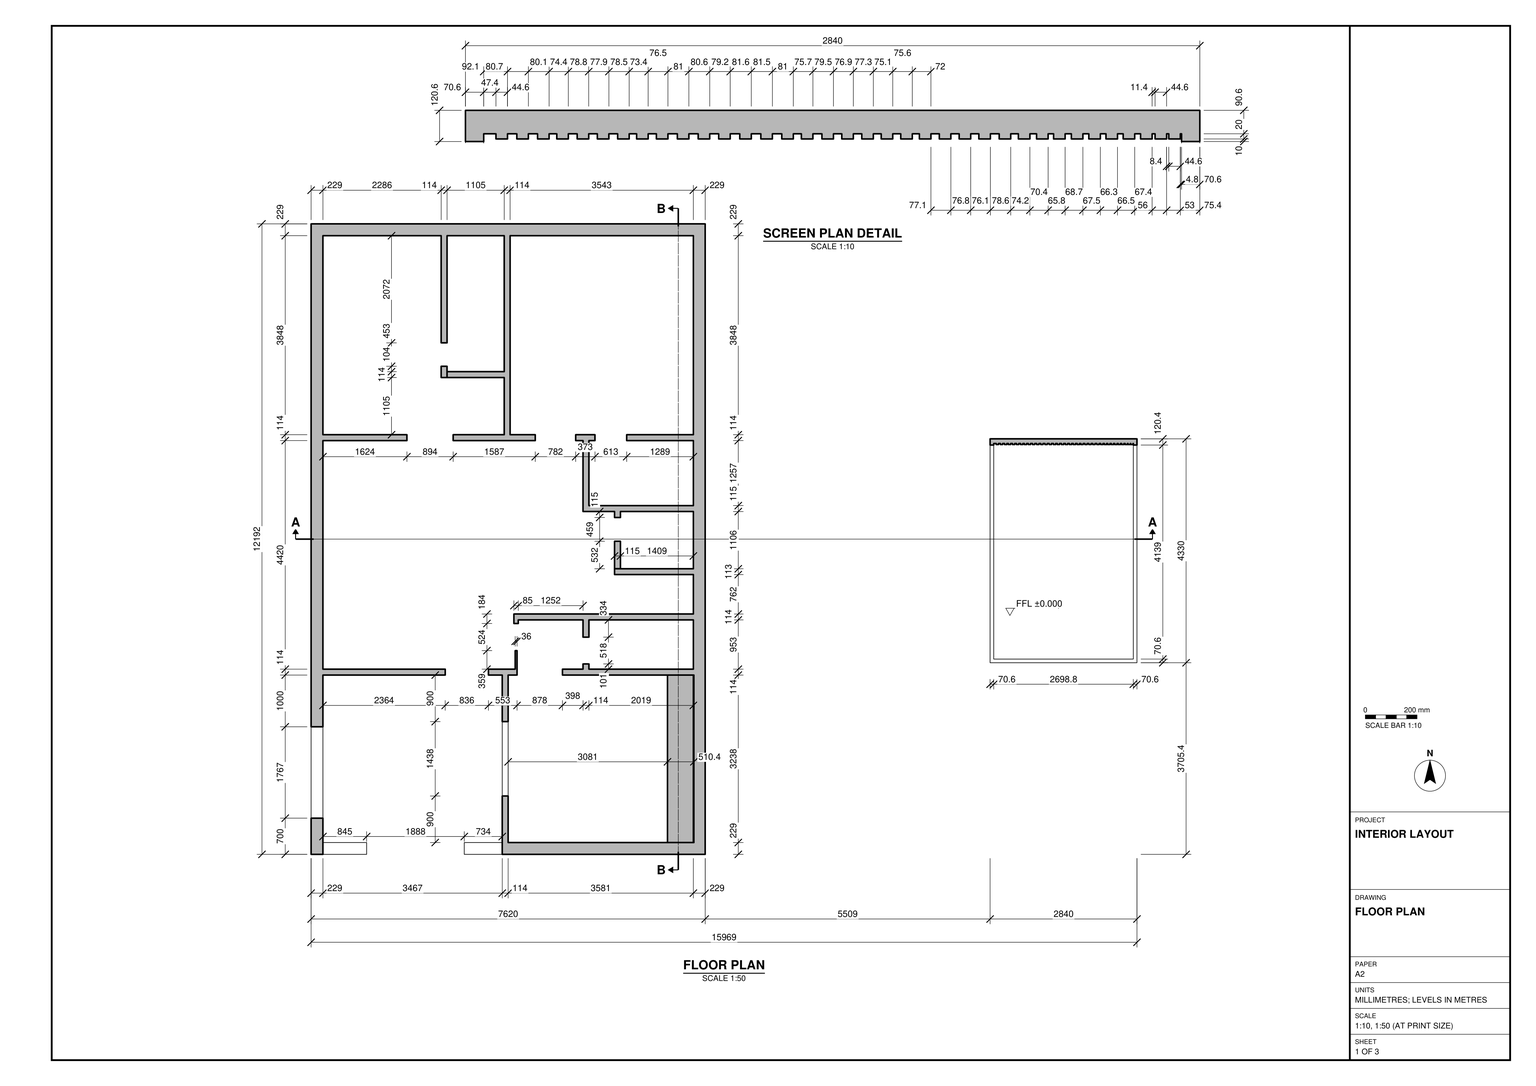
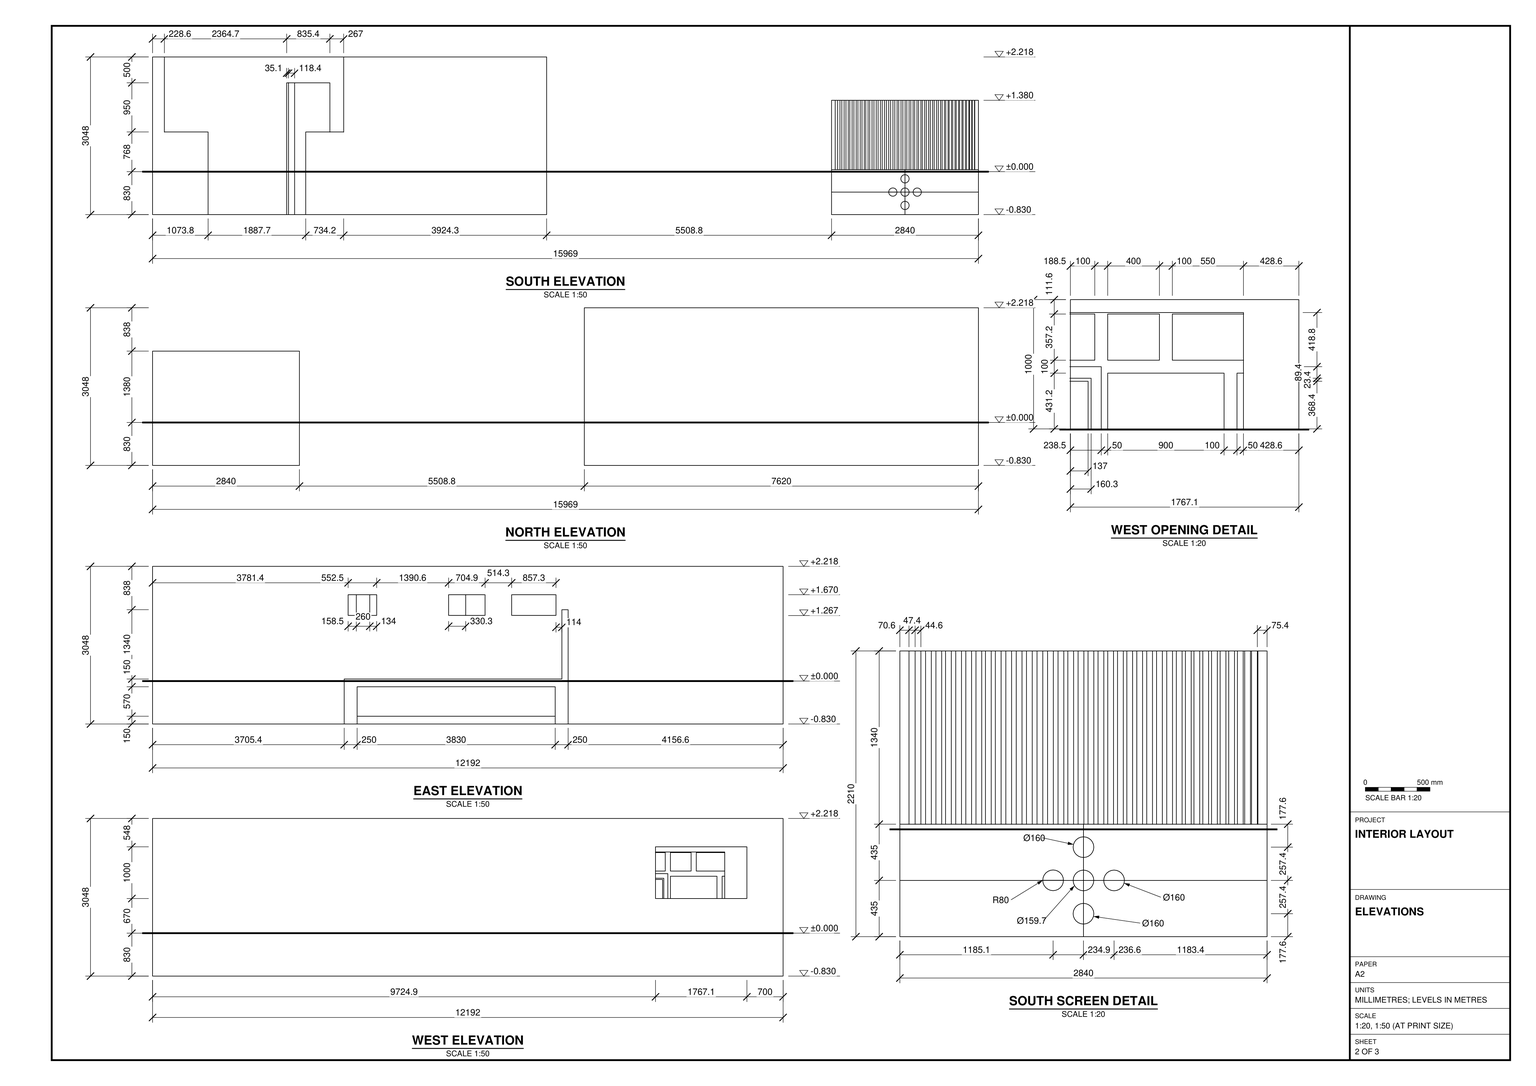
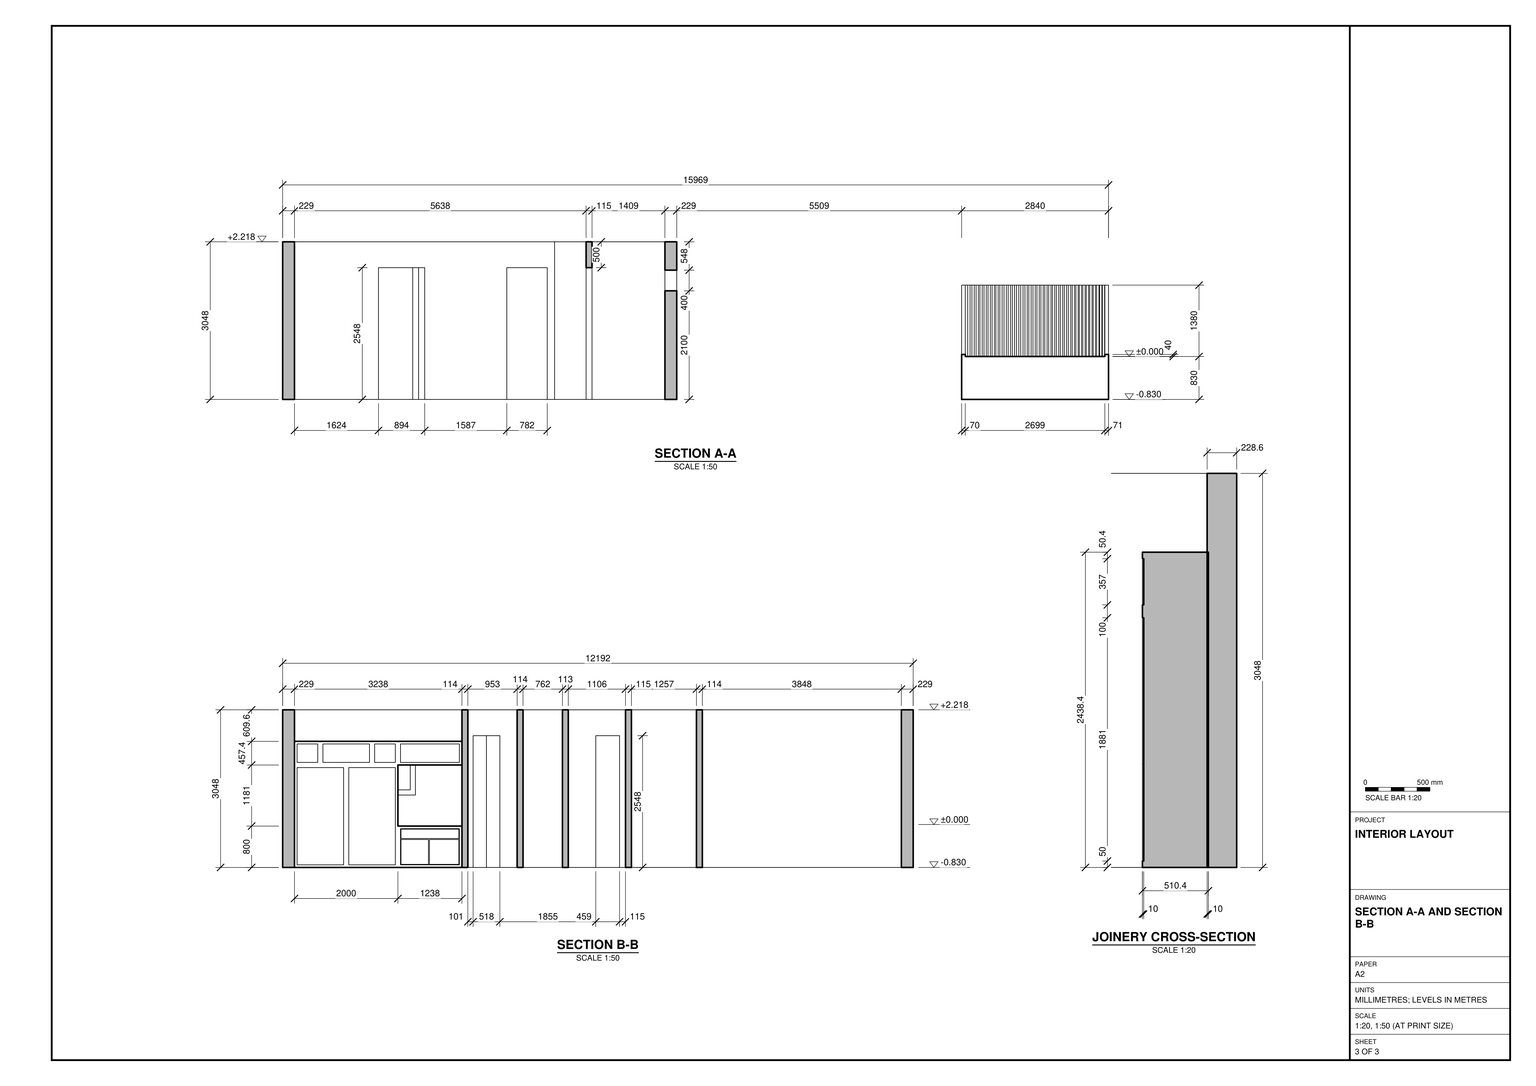
Build the interior in SketchUp from task_files/diagram_01.pdf. Work in millimetres. The complete layout, including the detached screen assembly, measures 15968.8 mm east to west, 12192 mm north to south and 3048 mm high. Use the single finished-floor datum marked ±0.000 (0 mm). The wall bases are at −830 mm and the wall heads at +2218 mm relative to this datum.

Set out the 7620 mm wide main shell from the floor plan. Follow the individual wall thicknesses: the perimeter walls are approximately 229 mm thick and most partitions are 114 mm thick. Keep the large central space open to the connecting passages, with the subdivided rooms to the north and the short partition returns to the east. Use the elevations for the exterior openings and section A-A for the interior doorway heads.

Fit the built-in storage against the east wall of the southeast room. Use section B-B for the arrangement of tall fronts, overhead compartments and the recessed bay with low storage. Include the bed, sofa and dining set as separate furniture pieces. Place the detached screen assembly east of the shell at the offsets shown in plan, and use the enlarged details for its vertical ribs and lower panel.

Make the shell elements and each furniture or joinery piece separate groups or components, and use components for repeated parts. Decor and loose items may be any suitable library components. Save one SketchUp model as output_files/interior_with_built_in_storage_and_detached_screen.skp.

# SketchUp Ruby script. Lengths in millimetres.
U = 1.mm
M = Sketchup.active_model
def pt(a) = Geom::Point3d.new(a.map { |v| v * U })
def face(e, loops, mat)
  f = e.add_face(loops[0].map { |a| pt(a) })
  loops[1..].each { |l| e.add_face(l.map { |a| pt(a) }).erase! }
  f.material = f.back_material = mat if mat
  f
end
# faces: each face lists its corners as indices into pts; further lists are holes
def faces(e, pts, list, mat = nil) = list.each { |f| face(e, (f[0].is_a?(Array) ? f : [f]).map { |l| l.map { |i| pts[i] } }, mat) }
# xy, xz, yz: faces in a plane at the given z, y or x. An outline is a flat list of corners, or four numbers for a rectangle; further outlines are holes
def ring(l) = l.size == 4 ? [[l[0], l[1]], [l[2], l[1]], [l[2], l[3]], [l[0], l[3]]] : l.each_slice(2).to_a
def flat(e, list, mat, &to3) = list.each { |f| face(e, (f[0].is_a?(Array) ? f : [f]).map { |l| ring(l).map { |u, v| to3.(u, v) } }, mat) }
def xy(e, z, list, mat = nil) = flat(e, list, mat) { |x, y| [x, y, z] }
def xz(e, y, list, mat = nil) = flat(e, list, mat) { |x, z| [x, y, z] }
def yz(e, x, list, mat = nil) = flat(e, list, mat) { |y, z| [x, y, z] }
def lines(e, pts, list) = list.each { |a, b| e.add_line(pt(pts[a]), pt(pts[b])) }
# prism: a flat outline (further loops are holes) pulled along v
def prism(e, loops, v, mat = nil)
  f = face(e, loops, mat); d = Geom::Vector3d.new(v.map { |x| x * U })
  f.pushpull(f.normal.samedirection?(d) ? d.length : -d.length)
end
def box(e, o, s, mat = nil) = prism(e, [[o, [o[0] + s[0], o[1], o[2]], [o[0] + s[0], o[1] + s[1], o[2]], [o[0], o[1] + s[1], o[2]]]], [0, 0, s[2]], mat)
def at(x, y, z, deg = 0) = Geom::Transformation.translation(pt([x, y, z])) * Geom::Transformation.rotation(ORIGIN, Z_AXIS, deg.degrees)
def axes(o, x, y, z) = Geom::Transformation.new([*x, 0, *y, 0, *z, 0, *pt(o).to_a, 1])
def part(name) = M.definitions.add(name)
# library, detail: a bought-in or finely detailed component or shape, given as its bounding box
def library(name, o, s) = part(name).tap { |d| box(d.entities, o, s) }
def detail(e, o, s) = box(e.add_group.entities, o, s)
def put(e, d, t, mat = nil) = e.add_instance(d, t).tap { |i| i.material = mat if mat }
def group(e, t, mat = nil) = e.add_group.tap { |g| g.transformation = t; g.material = mat if mat }.entities
root = M.entities
M.materials.add("[Color D01]").color = [255, 242, 204]
M.materials.add("[Color M09]").color = [0, 0, 0]
M.materials.add("[Mirror 01]").color = [185, 185, 185]
M.materials.add("[Translucent Glass Gray]").color = [128, 128, 128]
M.materials["[Translucent Glass Gray]"].alpha = 0.5
M.materials.add("[Wood Floor Parquet]").color = [145, 89, 39]
c1 = library("TINKU 1.dwg",[0,0,0],[7620,12192,0.1])
c2 = part("Built-in storage unit")
xy(c2.entities,0,[[0,0,510.4,3238.5]],"[Wood Floor Parquet]")
xy(c2.entities,50,[[0,50,10,950],[0,1050,10,1950],[0,2050,10,3188.5]],"[Wood Floor Parquet]")
xy(c2.entities,59.6,[[0,2059.6,10,2590.4],[0,2609.6,10,3178.9]],"[Wood Floor Parquet]")
xy(c2.entities,540.4,[[0,2059.6,10,2590.4],[0,2609.6,10,3178.9]],"[Wood Floor Parquet]")
xy(c2.entities,559.6,[[0,2059.6,10,2600],[0,2600,10,3178.9]],"[Wood Floor Parquet]")
xy(c2.entities,740.4,[[0,2059.6,10,3178.9]])
xy(c2.entities,750,[[0,2050,10,3188.5]],"[Wood Floor Parquet]")
xy(c2.entities,800,[[0,2000,420,3238.5]],"[Wood Floor Parquet]")
xy(c2.entities,915.2,[[420,2101.5,440,3094.8]],"[Color D01]")
xy(c2.entities,1868.4,[[420,2101.5,440,3094.8]],"[Color D01]")
xy(c2.entities,1931.2,[[0,50,10,500],[0,500,10,950],[0,1050,10,1500],[0,1500,10,1950]],"[Wood Floor Parquet]")
xy(c2.entities,1981.2,[[0,2000,420,3238.5]],"[Wood Floor Parquet]")
xy(c2.entities,2031.2,[[0,50,10,450],[0,550,10,1000],[0,1000,10,1450],[0,1550,10,1950],[0,2050,10,3188.5]],"[Wood Floor Parquet]")
xy(c2.entities,2388.4,[[0,50,10,450],[0,550,10,1450],[0,1550,10,1950],[0,2050,10,3188.5]],"[Wood Floor Parquet]")
xy(c2.entities,2438.4,[[0,0,510.4,3238.5]],"[Wood Floor Parquet]")
xz(c2.entities,0,[[0,0,510.4,2438.4]],"[Wood Floor Parquet]")
xz(c2.entities,50,[[0,50,10,1931.2],[0,2031.2,10,2388.4]],"[Wood Floor Parquet]")
xz(c2.entities,450,[[0,2031.2,10,2388.4]])
xz(c2.entities,550,[[0,2031.2,10,2388.4]],"[Wood Floor Parquet]")
xz(c2.entities,950,[[0,50,10,1931.2]],"[Wood Floor Parquet]")
xz(c2.entities,1050,[[0,50,10,1931.2]],"[Wood Floor Parquet]")
xz(c2.entities,1450,[[0,2031.2,10,2388.4]],"[Wood Floor Parquet]")
xz(c2.entities,1550,[[0,2031.2,10,2388.4]],"[Wood Floor Parquet]")
xz(c2.entities,1950,[[0,50,10,800],[0,800,10,1931.2],[0,2031.2,10,2388.4]],"[Wood Floor Parquet]")
xz(c2.entities,2000,[[0,800,420,1981.2]],"[Wood Floor Parquet]")
xz(c2.entities,2050,[[0,50,10,750],[0,2031.2,10,2388.4]],"[Wood Floor Parquet]")
xz(c2.entities,2059.6,[[0,59.6,10,540.4],[0,559.6,10,740.4]],"[Wood Floor Parquet]")
xz(c2.entities,2101.5,[[420,915.2,440,1868.4]],"[Color D01]")
xz(c2.entities,2590.4,[[0,59.6,10,540.4]],"[Wood Floor Parquet]")
xz(c2.entities,2609.6,[[0,59.6,10,540.4]],"[Wood Floor Parquet]")
xz(c2.entities,3094.8,[[420,915.2,440,1868.4]],"[Color D01]")
xz(c2.entities,3178.9,[[0,59.6,10,540.4],[0,559.6,10,740.4]],"[Wood Floor Parquet]")
xz(c2.entities,3188.5,[[0,50,10,750],[0,2031.2,10,2388.4]],"[Wood Floor Parquet]")
xz(c2.entities,3238.5,[[0,0,0,800,420,800,420,1981.2,0,1981.2,0,2438.4,510.4,2438.4,510.4,0]],"[Wood Floor Parquet]")
yz(c2.entities,0,[[2059.6,59.6,2590.4,540.4],[2609.6,59.6,3178.9,540.4],[2059.6,559.6,3178.9,740.4]],"[Translucent Glass Gray]")
yz(c2.entities,0,[[[0,0,0,2438.4,3238.5,2438.4,3238.5,1981.2,2000,1981.2,2000,800,3238.5,800,3238.5,0],[1050,50,1950,1931.2],[50,50,950,1931.2],[2050,50,3188.5,750],[2050,2031.2,3188.5,2388.4],[550,2031.2,1450,2388.4],[1550,2031.2,1950,2388.4],[50,2031.2,450,2388.4]]],"[Wood Floor Parquet]")
yz(c2.entities,10,[[50,50,950,1931.2],[1050,50,1950,1931.2],[50,2031.2,450,2388.4],[550,2031.2,1450,2388.4],[1550,2031.2,1950,2388.4],
  [2050,2031.2,3188.5,2388.4]],"[Translucent Glass Gray]")
yz(c2.entities,10,[[[2050,50,3188.5,750],[2609.6,59.6,3178.9,540.4],[2059.6,59.6,2590.4,540.4],[2059.6,559.6,3178.9,740.4]]],"[Wood Floor Parquet]")
yz(c2.entities,420,[[[2078.2,891.8,3118.2,1891.8],[2101.5,915.2,3094.8,1868.4]]],"[Color M09]")
yz(c2.entities,420,[[[2000,800,3238.5,1981.2],[2078.2,891.8,3118.2,1891.8]]],"[Wood Floor Parquet]")
yz(c2.entities,440,[[2101.5,915.2,3094.8,1868.4]],"[Mirror 01]")
yz(c2.entities,510.4,[[0,0,3238.5,2438.4]],"[Wood Floor Parquet]")
xy(root,0,[[0,0,0,12192,7620,12192,7620,0,2961.5,0,2961.5,228.6,7391.4,228.6,7391.4,11963.4,228.6,11963.4,228.6,228.6,1073.8,228.6,1073.8,0],[1073.8,0,2961.5,228.6],[3695.7,228.6,3695.7,3467.1,3428.7,3467.1,3428.7,3581.4,3982.2,3581.4,3982.2,3467.1,3810,3467.1,3810,228.6],[6891,228.6,7391.4,3467.1],[228.6,3467.1,2593.3,3581.4],
  [4860.1,3467.1,4860.1,3581.4,5257.8,3581.4,5257.8,3682.5,5372.1,3682.5,5372.1,3581.4,7391.4,3581.4,7391.4,3467.1],[3946.3,3581.4,3982.2,3939.9],[13128.8,3705.4,15968.8,8035.4],[5257.8,4199.9,5257.8,4533.9,4005.5,4533.9,4005.5,4463.8,3921.2,4463.8,3921.2,4648.2,7391.4,4648.2,7391.4,4533.9,5372.1,4533.9,5372.1,4199.9],[5867.4,5410.2,7391.4,5523.1],
  [5867.4,5524.5,5981.7,6054.8],[5867.4,6513.8,5867.4,6629.4,5257.8,6629.4,5257.8,8001,5116.2,8001,5116.2,8115.3,5488.7,8115.3,5488.7,8001,5372.1,8001,5372.1,6743.7,7391.4,6743.7,7391.4,6629.4,5981.7,6629.4,5981.7,6513.8],[228.6,8001,1852.7,8115.3],[2746.8,8001,2746.8,8115.3,3733.8,8115.3,3733.8,9220.2,2628.9,9220.2,2628.9,9334.5,3733.8,9334.5,3733.8,11963.4,3848.1,11963.4,3848.1,8115.3,4334.3,8115.3,4334.3,8001],[6102.1,8001,7391.4,8115.3],
  [2628.9,9220,3733.8,9220,2628.9,9220.2],[3733.8,9220,3733.8,9220.2,2628.9,9220.2],[2514.6,9220.2,2628.4,9438.2],[2514.6,9891.4,2628.9,11963.4]])
xy(root,830,[[13199.4,3776,15898.2,3776,15898.2,7944.8,15893.4,7944.8,15893.4,7924.8,15848.8,7924.8,15848.8,7944.8,15840.4,7944.8,15840.4,7924.8,15795.8,7924.8,15795.8,7944.8,15784.4,7944.8,15784.4,7924.8,15739.7,7924.8,15739.7,7944.8,15717,7944.8,15717,7924.8,15672.4,7924.8,15672.4,7944.8,15650.5,7944.8,15650.5,7924.8,15605.8,7924.8,15605.8,7944.8,15584.2,7944.8,15584.2,7924.8,15539.5,7924.8,15539.5,7944.8,15516.6,7944.8,15516.6,7924.8,15472,7924.8,15472,7944.8,15447.9,7944.8,15447.9,7924.8,15403.3,7924.8,15403.3,7944.8,15382.1,7944.8,15382.1,7924.8,15337.5,7924.8,15337.5,7944.8,15311.8,7944.8,15311.8,7924.8,15267.1,7924.8,15267.1,7944.8,15237.5,7944.8,15237.5,7924.8,15192.9,7924.8,15192.9,7944.8,15158.9,7944.8,15158.9,7924.8,15114.3,7924.8,15114.3,7944.8,15082.8,7944.8,15082.8,7924.8,15038.2,7924.8,15038.2,7944.8,15006,7944.8,15006,7924.8,14961.4,7924.8,14961.4,7944.8,14928.9,7944.8,14928.9,7924.8,14884.3,7924.8,14884.3,7944.8,14856.9,7944.8,14856.9,7924.8,14812.3,7924.8,14812.3,7944.8,14781.3,7944.8,14781.3,7924.8,14736.6,7924.8,14736.6,7944.8,14706.2,7944.8,14706.2,7924.8,14661.6,7924.8,14661.6,7944.8,14628.9,7944.8,14628.9,7924.8,14584.3,7924.8,14584.3,7944.8,14552,7944.8,14552,7924.8,14507.4,7924.8,14507.4,7944.8,14472.5,7944.8,14472.5,7924.8,14427.9,7924.8,14427.9,7944.8,14396.8,7944.8,14396.8,7924.8,14352.2,7924.8,14352.2,7944.8,14315.8,7944.8,14315.8,7924.8,14271.2,7924.8,14271.2,7944.8,14234.3,7944.8,14234.3,7924.8,14189.7,7924.8,14189.7,7944.8,14152.7,7944.8,14152.7,7924.8,14108.1,7924.8,14108.1,7944.8,14073.5,7944.8,14073.5,7924.8,14028.9,7924.8,14028.9,7944.8,13992.9,7944.8,13992.9,7924.8,13948.3,7924.8,13948.3,7944.8,13911.9,7944.8,13911.9,7924.8,13867.3,7924.8,13867.3,7944.8,13835.4,7944.8,13835.4,7924.8,13790.8,7924.8,13790.8,7944.8,13762,7944.8,13762,7924.8,13717.4,7924.8,13717.4,7944.8,13683.5,7944.8,13683.5,7924.8,13638.8,7924.8,13638.8,7944.8,13605.5,7944.8,13605.5,7924.8,13560.9,7924.8,13560.9,7944.8,13526.7,7944.8,13526.7,7924.8,13482.1,7924.8,13482.1,7944.8,13452.3,7944.8,13452.3,7924.8,13407.6,7924.8,13407.6,7944.8,13372.2,7944.8,13372.2,7924.8,13327.6,7924.8,13327.6,7944.8,13291.5,7944.8,13291.5,7924.8,13246.8,7924.8,13246.8,7944.8,13199.4,7944.8]])
xy(root,870,[[13128.8,3705.4,15968.8,3705.4,15968.8,7914.8,15898.2,7914.8,15898.2,3776,13199.4,3776,13199.4,7914.8,13128.8,7914.8]])
xy(root,1400,[[3695.7,1128.6,3810,2567.1]])
xy(root,1500,[[0,700,228.6,2467.1]])
xy(root,1598,[[228.6,0,1073.8,228.6],[2961.5,0,3695.7,228.6]])
xy(root,2100,[[7391.4,3781.4,7620,4333.9],[7391.4,5724.5,7620,6429.4],[7391.4,6943.7,7620,7801]])
xy(root,2210,[[13128.8,7914.8,13199.4,7914.8,13199.4,7944.8,13246.8,7944.8,13246.8,7924.8,13291.5,7924.8,13291.5,7944.8,13327.6,7944.8,13327.6,7924.8,13372.2,7924.8,13372.2,7944.8,13407.6,7944.8,13407.6,7924.8,13452.3,7924.8,13452.3,7944.8,13482.1,7944.8,13482.1,7924.8,13526.7,7924.8,13526.7,7944.8,13560.9,7944.8,13560.9,7924.8,13605.5,7924.8,13605.5,7944.8,13638.8,7944.8,13638.8,7924.8,13683.5,7924.8,13683.5,7944.8,13717.4,7944.8,13717.4,7924.8,13762,7924.8,13762,7944.8,13790.8,7944.8,13790.8,7924.8,13835.4,7924.8,13835.4,7944.8,13867.3,7944.8,13867.3,7924.8,13911.9,7924.8,13911.9,7944.8,13948.3,7944.8,13948.3,7924.8,13992.9,7924.8,13992.9,7944.8,14028.9,7944.8,14028.9,7924.8,14073.5,7924.8,14073.5,7944.8,14108.1,7944.8,14108.1,7924.8,14152.7,7924.8,14152.7,7944.8,14189.7,7944.8,14189.7,7924.8,14234.3,7924.8,14234.3,7944.8,14271.2,7944.8,14271.2,7924.8,14315.8,7924.8,14315.8,7944.8,14352.2,7944.8,14352.2,7924.8,14396.8,7924.8,14396.8,7944.8,14427.9,7944.8,14427.9,7924.8,14472.5,7924.8,14472.5,7944.8,14507.4,7944.8,14507.4,7924.8,14552,7924.8,14552,7944.8,14584.3,7944.8,14584.3,7924.8,14628.9,7924.8,14628.9,7944.8,14661.6,7944.8,14661.6,7924.8,14706.2,7924.8,14706.2,7944.8,14736.6,7944.8,14736.6,7924.8,14781.3,7924.8,14781.3,7944.8,14812.3,7944.8,14812.3,7924.8,14856.9,7924.8,14856.9,7944.8,14884.3,7944.8,14884.3,7924.8,14928.9,7924.8,14928.9,7944.8,14961.4,7944.8,14961.4,7924.8,15006,7924.8,15006,7944.8,15038.2,7944.8,15038.2,7924.8,15082.8,7924.8,15082.8,7944.8,15114.3,7944.8,15114.3,7924.8,15158.9,7924.8,15158.9,7944.8,15192.9,7944.8,15192.9,7924.8,15237.5,7924.8,15237.5,7944.8,15267.1,7944.8,15267.1,7924.8,15311.8,7924.8,15311.8,7944.8,15337.5,7944.8,15337.5,7924.8,15382.1,7924.8,15382.1,7944.8,15403.3,7944.8,15403.3,7924.8,15447.9,7924.8,15447.9,7944.8,15472,7944.8,15472,7924.8,15516.6,7924.8,15516.6,7944.8,15539.5,7944.8,15539.5,7924.8,15584.2,7924.8,15584.2,7944.8,15605.8,7944.8,15605.8,7924.8,15650.5,7924.8,15650.5,7944.8,15672.4,7944.8,15672.4,7924.8,15717,7924.8,15717,7944.8,15739.7,7944.8,15739.7,7924.8,15784.4,7924.8,15784.4,7944.8,15795.8,7944.8,15795.8,7924.8,15840.4,7924.8,15840.4,7944.8,15848.8,7944.8,15848.8,7924.8,15893.4,7924.8,15893.4,7944.8,15898.2,7944.8,15898.2,7914.8,15968.8,7914.8,15968.8,8035.4,13128.8,8035.4]])
xy(root,2400,[[3695.7,1128.6,3810,2567.1]])
xy(root,2500,[[0,700,228.6,2467.1],[7391.4,3781.4,7620,4333.9],[7391.4,5724.5,7620,6429.4],[7391.4,6943.7,7620,7801]])
xy(root,2548,[[2593.3,3467.1,3428.7,3581.4],[3982.2,3467.1,4860.1,3581.4],[5257.8,3682.5,5372.1,4199.9],[5867.4,6054.8,5981.7,6513.8],[1852.7,8001,2746.8,8115.3],
  [4334.3,8001,5116.2,8115.3],[5488.7,8001,6102.1,8115.3],[2514.6,9438.2,2628.4,9891.4]])
xy(root,3048,[[[0,0,228.6,0,228.6,3467.1,3695.7,3467.1,3695.7,0,7620,0,7620,12192,0,12192],[228.6,3581.4,228.6,8001,5257.8,8001,5257.8,6629.4,5867.4,6629.4,5867.4,5524.5,5981.7,5524.5,5981.7,6629.4,7391.4,6629.4,7391.4,5523.1,5867.4,5523.1,5867.4,5410.2,7391.4,5410.2,7391.4,4648.2,3921.2,4648.2,3921.2,4463.8,4005.5,4463.8,4005.5,4533.9,5257.8,4533.9,5257.8,3581.4,3982.2,3581.4,3982.2,3939.9,3946.3,3939.9,3946.3,3581.4],[3848.1,8115.3,7391.4,11963.4],[228.6,8115.3,228.6,11963.4,2514.6,11963.4,2514.6,9220.2,2628.4,9220.2,2628.4,9891.4,2628.9,9891.4,2628.9,11963.4,3733.8,11963.4,3733.8,9334.5,2628.9,9334.5,2628.9,9220.2,3733.8,9220.2,3733.8,8115.3],[3810,228.6,7391.4,3467.1],[5372.1,6743.7,7391.4,8001],[5372.1,3581.4,7391.4,4533.9]]])
xz(root,0,[[0,0,1073.8,0,1073.8,1598,228.6,1598,228.6,3048,0,3048],[2961.5,0,7620,0,7620,3048,3695.7,3048,3695.7,1598,2961.5,1598]])
xz(root,228.6,[[228.6,0,1073.8,1598],[2961.5,0,3695.7,1598],[3810,0,7391.4,3048]])
xz(root,700,[[0,1500,228.6,2500]])
xz(root,1128.6,[[3695.7,1400,3810,2400]])
xz(root,2467.1,[[0,1500,228.6,2500]])
xz(root,2567.1,[[3695.7,1400,3810,2400]])
xz(root,3467.1,[[228.6,0,2593.3,0,2593.3,2548,3428.7,2548,3428.7,0,3695.7,0,3695.7,3048,228.6,3048],[3810,0,3982.2,0,3982.2,2548,4860.1,2548,4860.1,0,7391.4,0,7391.4,3048,3810,3048]])
xz(root,3581.4,[[228.6,0,228.6,3048,3946.3,3048,3946.3,0,3428.7,0,3428.7,2548,2593.3,2548,2593.3,0],[4860.1,0,4860.1,2548,3982.2,2548,3982.2,3048,5257.8,3048,5257.8,0],[5372.1,0,7391.4,3048]])
xz(root,3682.5,[[5257.8,0,5372.1,2548]])
xz(root,3705.4,[[13128.8,0,14548.8,0,14548.8,97.6,14528.1,100.3,14508.8,108.3,14492.3,121,14479.6,137.6,14471.6,156.9,14468.8,177.6,14471.6,198.3,14479.6,217.6,14492.3,234.1,14508.8,246.8,14528.1,254.8,14548.8,257.6,14548.8,355.1,14528.2,357.8,14508.9,365.8,14492.4,378.5,14479.7,395.1,14471.7,414.3,14469,435,14393.8,435,14391.2,415.2,14383.2,395.9,14370.5,379.4,14354,366.7,14334.7,358.7,14314,355.9,14293.2,358.7,14274,366.7,14257.4,379.4,14244.7,395.9,14236.7,415.2,14234.1,435,13128.8,435],[14548.8,0,15968.8,0,15968.8,435,14865.5,435,14862.7,414.3,14854.7,395,14842,378.4,14825.5,365.7,14806.2,357.7,14785.5,355,14764.8,357.7,14745.5,365.7,14728.9,378.4,14716.2,395,14708.2,414.3,14705.5,435,14628.7,435,14626,414.3,14618,395.1,14605.3,378.5,14588.8,365.8,14569.5,357.8,14548.8,355.1,14548.8,257.6,14569.5,254.8,14588.8,246.8,14605.4,234.1,14618.1,217.6,14626.1,198.3,14628.8,177.6,14626.1,156.9,14618.1,137.6,14605.4,121,14588.8,108.3,14569.5,100.3,14548.8,97.6],[14548.8,97.6,14548.8,257.6,14528.1,254.8,14508.8,246.8,14492.3,234.1,14479.6,217.6,14471.6,198.3,14468.8,177.6,14471.6,156.9,14479.6,137.6,14492.3,121,14508.8,108.3,14528.1,100.3],[14548.8,97.6,14569.5,100.3,14588.8,108.3,14605.4,121,14618.1,137.6,14626.1,156.9,14628.8,177.6,14626.1,198.3,14618.1,217.6,14605.4,234.1,14588.8,246.8,14569.5,254.8,14548.8,257.6],[14785.5,355,14806.2,357.7,14825.5,365.7,14842,378.4,14854.7,395,14862.7,414.3,14865.5,435,14705.5,435,14708.2,414.3,14716.2,395,14728.9,378.4,14745.5,365.7,14764.8,357.7],
  [14548.8,355.1,14548.8,435,14469,435,14471.7,414.3,14479.7,395.1,14492.4,378.5,14508.9,365.8,14528.2,357.8],[14548.8,355.1,14569.5,357.8,14588.8,365.8,14605.3,378.5,14618,395.1,14626,414.3,14628.7,435,14548.8,435],[14314,355.9,14334.7,358.7,14354,366.7,14370.5,379.4,14383.2,395.9,14391.2,415.2,14393.8,435,14234.1,435,14236.7,415.2,14244.7,395.9,14257.4,379.4,14274,366.7,14293.2,358.7],[13128.8,435,14234.1,435,14234,435.9,14236.7,456.6,14244.7,475.9,14257.4,492.5,14274,505.2,14293.2,513.2,14314,515.9,14334.7,513.2,14354,505.2,14370.5,492.5,14383.2,475.9,14391.2,456.6,14394,435.9,14393.8,435,14469,435,14471.7,455.7,14479.7,474.9,14492.4,491.5,14508.9,504.2,14528.2,512.2,14548.8,514.9,14548.8,612.4,14528.1,615.2,14508.8,623.2,14492.3,635.9,14479.6,652.4,14471.6,671.7,14468.8,692.4,14471.6,713.1,14479.6,732.4,14492.3,749,14508.8,761.7,14528.1,769.7,14548.8,772.4,14548.8,870,13128.8,870],[14234.1,435,14393.8,435,14394,435.9,14234,435.9],
  [14469,435,14548.8,435,14548.8,514.9,14528.2,512.2,14508.9,504.2,14492.4,491.5,14479.7,474.9,14471.7,455.7],[14548.8,435,14628.7,435,14626,455.7,14618,474.9,14605.3,491.5,14588.8,504.2,14569.5,512.2,14548.8,514.9],[14628.7,435,14705.5,435,14708.2,455.7,14716.2,475,14728.9,491.6,14745.5,504.3,14764.8,512.3,14785.5,515,14806.2,512.3,14825.5,504.3,14842,491.6,14854.7,475,14862.7,455.7,14865.5,435,15968.8,435,15968.8,870,14548.8,870,14548.8,772.4,14569.5,769.7,14588.8,761.7,14605.4,749,14618.1,732.4,14626.1,713.1,14628.8,692.4,14626.1,671.7,14618.1,652.4,14605.4,635.9,14588.8,623.2,14569.5,615.2,14548.8,612.4,14548.8,514.9,14569.5,512.2,14588.8,504.2,14605.3,491.5,14618,474.9,14626,455.7],[14705.5,435,14865.5,435,14862.7,455.7,14854.7,475,14842,491.6,14825.5,504.3,14806.2,512.3,14785.5,515,14764.8,512.3,14745.5,504.3,14728.9,491.6,14716.2,475,14708.2,455.7],[14234,435.9,14394,435.9,14391.2,456.6,14383.2,475.9,14370.5,492.5,14354,505.2,14334.7,513.2,14314,515.9,14293.2,513.2,14274,505.2,14257.4,492.5,14244.7,475.9,14236.7,456.6],
  [14548.8,612.4,14548.8,772.4,14528.1,769.7,14508.8,761.7,14492.3,749,14479.6,732.4,14471.6,713.1,14468.8,692.4,14471.6,671.7,14479.6,652.4,14492.3,635.9,14508.8,623.2,14528.1,615.2],[14548.8,612.4,14569.5,615.2,14588.8,623.2,14605.4,635.9,14618.1,652.4,14626.1,671.7,14628.8,692.4,14626.1,713.1,14618.1,732.4,14605.4,749,14588.8,761.7,14569.5,769.7,14548.8,772.4]])
xz(root,3776,[[13199.4,830,14548.8,870],[14548.8,830,15898.2,870]])
xz(root,3781.4,[[7391.4,2100,7620,2500]])
xz(root,3939.9,[[3946.3,0,3982.2,3048]])
xz(root,4199.9,[[5257.8,0,5372.1,2548]])
xz(root,4333.9,[[7391.4,2100,7620,2500]])
xz(root,4463.8,[[3921.2,0,4005.5,3048]])
xz(root,4533.9,[[4005.5,0,5257.8,3048],[5372.1,0,7391.4,3048]])
xz(root,4648.2,[[3921.2,0,7391.4,3048]])
xz(root,5410.2,[[5867.4,0,7391.4,3048]])
xz(root,5523.1,[[5867.4,0,7391.4,3048]])
xz(root,5524.5,[[5867.4,0,5981.7,3048]])
xz(root,5724.5,[[7391.4,2100,7620,2500]])
xz(root,6054.8,[[5867.4,0,5981.7,2548]])
xz(root,6429.4,[[7391.4,2100,7620,2500]])
xz(root,6513.8,[[5867.4,0,5981.7,2548]])
xz(root,6629.4,[[5257.8,0,5867.4,3048],[5981.7,0,7391.4,3048]])
xz(root,6743.7,[[5372.1,0,7391.4,3048]])
xz(root,6943.7,[[7391.4,2100,7620,2500]])
xz(root,7801,[[7391.4,2100,7620,2500]])
xz(root,7914.8,[[13128.8,870,13199.4,2210],[15898.2,870,15968.8,2210]])
xz(root,7924.8,[[13246.8,830,13291.5,2210],[13327.6,830,13372.2,2210],[13407.6,830,13452.3,2210],[13482.1,830,13526.7,2210],[13560.9,830,13605.5,2210],
  [13638.8,830,13683.5,2210],[13717.4,830,13762,2210],[13790.8,830,13835.4,2210],[13867.3,830,13911.9,2210],[13948.3,830,13992.9,2210],
  [14028.9,830,14073.5,2210],[14108.1,830,14152.7,2210],[14189.7,830,14234.3,2210],[14271.2,830,14315.8,2210],[14352.2,830,14396.8,2210],
  [14427.9,830,14472.5,2210],[14507.4,830,14552,2210],[14584.3,830,14628.9,2210],[14661.6,830,14706.2,2210],[14736.6,830,14781.3,2210],
  [14812.3,830,14856.9,2210],[14884.3,830,14928.9,2210],[14961.4,830,15006,2210],[15038.2,830,15082.8,2210],[15114.3,830,15158.9,2210],
  [15192.9,830,15237.5,2210],[15267.1,830,15311.8,2210],[15337.5,830,15382.1,2210],[15403.3,830,15447.9,2210],[15472,830,15516.6,2210],
  [15539.5,830,15584.2,2210],[15605.8,830,15650.5,2210],[15672.4,830,15717,2210],[15739.7,830,15784.4,2210],[15795.8,830,15840.4,2210],
  [15848.8,830,15893.4,2210]])
xz(root,7944.8,[[13199.4,830,13246.8,2210],[13291.5,830,13327.6,2210],[13372.2,830,13407.6,2210],[13452.3,830,13482.1,2210],[13526.7,830,13560.9,2210],
  [13605.5,830,13638.8,2210],[13683.5,830,13717.4,2210],[13762,830,13790.8,2210],[13835.4,830,13867.3,2210],[13911.9,830,13948.3,2210],
  [13992.9,830,14028.9,2210],[14073.5,830,14108.1,2210],[14152.7,830,14189.7,2210],[14234.3,830,14271.2,2210],[14315.8,830,14352.2,2210],
  [14396.8,830,14427.9,2210],[14472.5,830,14507.4,2210],[14552,830,14584.3,2210],[14628.9,830,14661.6,2210],[14706.2,830,14736.6,2210],
  [14781.3,830,14812.3,2210],[14856.9,830,14884.3,2210],[14928.9,830,14961.4,2210],[15006,830,15038.2,2210],[15082.8,830,15114.3,2210],
  [15158.9,830,15192.9,2210],[15237.5,830,15267.1,2210],[15311.8,830,15337.5,2210],[15382.1,830,15403.3,2210],[15447.9,830,15472,2210],
  [15516.6,830,15539.5,2210],[15584.2,830,15605.8,2210],[15650.5,830,15672.4,2210],[15717,830,15739.7,2210],[15784.4,830,15795.8,2210],
  [15840.4,830,15848.8,2210],[15893.4,830,15898.2,2210]])
xz(root,8001,[[228.6,0,1852.7,0,1852.7,2548,2746.8,2548,2746.8,0,4334.3,0,4334.3,2548,5116.2,2548,5116.2,0,5257.8,0,5257.8,3048,228.6,3048],[5372.1,0,5488.7,0,5488.7,2548,6102.1,2548,6102.1,0,7391.4,0,7391.4,3048,5372.1,3048]])
xz(root,8035.4,[[13128.8,0,15968.8,2210]])
xz(root,8115.3,[[228.6,0,228.6,3048,3733.8,3048,3733.8,0,2746.8,0,2746.8,2548,1852.7,2548,1852.7,0],[3848.1,0,3848.1,3048,7391.4,3048,7391.4,0,6102.1,0,6102.1,2548,5488.7,2548,5488.7,0,5116.2,0,5116.2,2548,4334.3,2548,4334.3,0]])
xz(root,9220.2,[[2514.6,0,2628.4,3048],[2628.9,0,3733.8,3048]])
xz(root,9334.5,[[2628.9,0,3733.8,3048]])
xz(root,9438.2,[[2514.6,0,2628.4,2548]])
xz(root,9891.4,[[2514.6,0,2628.9,0,2628.9,3048,2628.4,3048,2628.4,2548,2514.6,2548]])
xz(root,11963.4,[[228.6,0,2514.6,3048],[2628.9,0,3733.8,3048],[3848.1,0,7391.4,3048]])
xz(root,12192,[[0,0,7620,3048]])
yz(root,0,[[[0,0,12192,3048],[700,1500,2467.1,2500]]])
yz(root,228.6,[[[228.6,0,3467.1,0,3467.1,3048,0,3048,0,1598,228.6,1598],[700,1500,2467.1,2500]],[3581.4,0,8001,3048],[8115.3,0,11963.4,3048]])
yz(root,1073.8,[[0,0,228.6,1598]])
yz(root,1852.7,[[8001,0,8115.3,2548]])
yz(root,2514.6,[[9220.2,0,9220.2,3048,11963.4,3048,11963.4,0,9891.4,0,9891.4,2548,9438.2,2548,9438.2,0]])
yz(root,2593.3,[[3467.1,0,3581.4,2548]])
yz(root,2628.4,[[9220.2,0,9438.2,0,9438.2,2548,9891.4,2548,9891.4,3048,9220.2,3048]])
yz(root,2628.9,[[9220.2,0,9334.5,3048],[9891.4,0,11963.4,3048]])
yz(root,2746.8,[[8001,0,8115.3,2548]])
yz(root,2961.5,[[0,0,228.6,1598]])
yz(root,3428.7,[[3467.1,0,3581.4,2548]])
yz(root,3695.7,[[[228.6,0,228.6,1598,0,1598,0,3048,3467.1,3048,3467.1,0],[1128.6,1400,2567.1,2400]]])
yz(root,3733.8,[[8115.3,0,9220,3048],[9220,0,9220.2,3048],[9334.5,0,9335.1,3048],[9335.1,0,11963.4,3048]])
yz(root,3810,[[[228.6,0,3467.1,3048],[1128.6,1400,2567.1,2400]]])
yz(root,3848.1,[[8115.3,0,11963.4,3048]])
yz(root,3921.2,[[4463.8,0,4648.2,3048]])
yz(root,3946.3,[[3581.4,0,3939.9,3048]])
yz(root,3982.2,[[3467.1,0,3939.9,0,3939.9,3048,3581.4,3048,3581.4,2548,3467.1,2548]])
yz(root,4005.5,[[4463.8,0,4533.9,3048]])
yz(root,4334.3,[[8001,0,8115.3,2548]])
yz(root,4860.1,[[3467.1,0,3581.4,2548]])
yz(root,5116.2,[[8001,0,8115.3,2548]])
yz(root,5257.8,[[3581.4,0,3581.4,3048,4533.9,3048,4533.9,0,4199.9,0,4199.9,2548,3682.5,2548,3682.5,0],[6629.4,0,8001,3048]])
yz(root,5372.1,[[3581.4,0,3682.5,0,3682.5,2548,4199.9,2548,4199.9,0,4533.9,0,4533.9,3048,3581.4,3048],[6743.7,0,8001,3048]])
yz(root,5488.7,[[8001,0,8115.3,2548]])
yz(root,5867.4,[[5410.2,0,5523.1,3048],[5524.5,0,5524.5,3048,6629.4,3048,6629.4,0,6513.8,0,6513.8,2548,6054.8,2548,6054.8,0]])
yz(root,5981.7,[[5524.5,0,6054.8,0,6054.8,2548,6513.8,2548,6513.8,0,6629.4,0,6629.4,3048,5524.5,3048]])
yz(root,6102.1,[[8001,0,8115.3,2548]])
yz(root,7391.4,[[228.6,0,3467.1,3048],[[3581.4,0,4533.9,3048],[3781.4,2100,4333.9,2500]],[4648.2,0,5410.2,3048],[5523.1,0,5524.5,3048],[[5524.5,0,6629.4,3048],[5724.5,2100,6429.4,2500]],
  [[6743.7,0,8001,3048],[6943.7,2100,7801,2500]],[8115.3,0,11963.4,3048]])
yz(root,7620,[[[0,0,12192,3048],[6943.7,2100,7801,2500],[5724.5,2100,6429.4,2500],[3781.4,2100,4333.9,2500]]])
yz(root,13128.8,[[3705.4,0,3705.4,870,7914.8,870,7914.8,2210,8035.4,2210,8035.4,0,7785.4,0,7785.4,720,3955.4,720,3955.4,0],[3955.4,0,7785.4,150],[3955.4,150,7785.4,720]])
yz(root,13199.4,[[3776,830,7914.8,870],[7914.8,830,7944.8,2210]])
yz(root,13246.8,[[7924.8,830,7944.8,2210]])
yz(root,13291.5,[[7924.8,830,7944.8,2210]])
yz(root,13327.6,[[7924.8,830,7944.8,2210]])
yz(root,13372.2,[[7924.8,830,7944.8,2210]])
yz(root,13407.6,[[7924.8,830,7944.8,2210]])
yz(root,13452.3,[[7924.8,830,7944.8,2210]])
yz(root,13482.1,[[7924.8,830,7944.8,2210]])
yz(root,13526.7,[[7924.8,830,7944.8,2210]])
yz(root,13560.9,[[7924.8,830,7944.8,2210]])
yz(root,13605.5,[[7924.8,830,7944.8,2210]])
yz(root,13638.8,[[7924.8,830,7944.8,2210]])
yz(root,13683.5,[[7924.8,830,7944.8,2210]])
yz(root,13717.4,[[7924.8,830,7944.8,2210]])
yz(root,13762,[[7924.8,830,7944.8,2210]])
yz(root,13790.8,[[7924.8,830,7944.8,2210]])
yz(root,13835.4,[[7924.8,830,7944.8,2210]])
yz(root,13867.3,[[7924.8,830,7944.8,2210]])
yz(root,13911.9,[[7924.8,830,7944.8,2210]])
yz(root,13948.3,[[7924.8,830,7944.8,2210]])
yz(root,13992.9,[[7924.8,830,7944.8,2210]])
yz(root,14028.9,[[7924.8,830,7944.8,2210]])
yz(root,14073.5,[[7924.8,830,7944.8,2210]])
yz(root,14108.1,[[7924.8,830,7944.8,2210]])
yz(root,14152.7,[[7924.8,830,7944.8,2210]])
yz(root,14189.7,[[7924.8,830,7944.8,2210]])
yz(root,14234.3,[[7924.8,830,7944.8,2210]])
yz(root,14271.2,[[7924.8,830,7944.8,2210]])
yz(root,14315.8,[[7924.8,830,7944.8,2210]])
yz(root,14352.2,[[7924.8,830,7944.8,2210]])
yz(root,14396.8,[[7924.8,830,7944.8,2210]])
yz(root,14427.9,[[7924.8,830,7944.8,2210]])
yz(root,14472.5,[[7924.8,830,7944.8,2210]])
yz(root,14507.4,[[7924.8,830,7944.8,2210]])
yz(root,14552,[[7924.8,830,7944.8,2210]])
yz(root,14584.3,[[7924.8,830,7944.8,2210]])
yz(root,14628.9,[[7924.8,830,7944.8,2210]])
yz(root,14661.6,[[7924.8,830,7944.8,2210]])
yz(root,14706.2,[[7924.8,830,7944.8,2210]])
yz(root,14736.6,[[7924.8,830,7944.8,2210]])
yz(root,14781.3,[[7924.8,830,7944.8,2210]])
yz(root,14812.3,[[7924.8,830,7944.8,2210]])
yz(root,14856.9,[[7924.8,830,7944.8,2210]])
yz(root,14884.3,[[7924.8,830,7944.8,2210]])
yz(root,14928.9,[[7924.8,830,7944.8,2210]])
yz(root,14961.4,[[7924.8,830,7944.8,2210]])
yz(root,15006,[[7924.8,830,7944.8,2210]])
yz(root,15038.2,[[7924.8,830,7944.8,2210]])
yz(root,15082.8,[[7924.8,830,7944.8,2210]])
yz(root,15114.3,[[7924.8,830,7944.8,2210]])
yz(root,15158.9,[[7924.8,830,7944.8,2210]])
yz(root,15192.9,[[7924.8,830,7944.8,2210]])
yz(root,15237.5,[[7924.8,830,7944.8,2210]])
yz(root,15267.1,[[7924.8,830,7944.8,2210]])
yz(root,15311.8,[[7924.8,830,7944.8,2210]])
yz(root,15337.5,[[7924.8,830,7944.8,2210]])
yz(root,15382.1,[[7924.8,830,7944.8,2210]])
yz(root,15403.3,[[7924.8,830,7944.8,2210]])
yz(root,15447.9,[[7924.8,830,7944.8,2210]])
yz(root,15472,[[7924.8,830,7944.8,2210]])
yz(root,15516.6,[[7924.8,830,7944.8,2210]])
yz(root,15539.5,[[7924.8,830,7944.8,2210]])
yz(root,15584.2,[[7924.8,830,7944.8,2210]])
yz(root,15605.8,[[7924.8,830,7944.8,2210]])
yz(root,15650.5,[[7924.8,830,7944.8,2210]])
yz(root,15672.4,[[7924.8,830,7944.8,2210]])
yz(root,15717,[[7924.8,830,7944.8,2210]])
yz(root,15739.7,[[7924.8,830,7944.8,2210]])
yz(root,15784.4,[[7924.8,830,7944.8,2210]])
yz(root,15795.8,[[7924.8,830,7944.8,2210]])
yz(root,15840.4,[[7924.8,830,7944.8,2210]])
yz(root,15848.8,[[7924.8,830,7944.8,2210]])
yz(root,15893.4,[[7924.8,830,7944.8,2210]])
yz(root,15898.2,[[3776,830,7914.8,870],[7914.8,830,7944.8,2210]])
yz(root,15968.8,[[3705.4,0,3955.4,0,3955.4,720,7785.4,720,7785.4,0,8035.4,0,8035.4,2210,7914.8,2210,7914.8,870,3705.4,870],[3955.4,0,7785.4,150],[3955.4,150,7785.4,720]])
p = [[228.6,11963.4,0],[228.6,11970.3,0],[5372.1,8001,0],[5369.3,8001,0],[5981.7,5524.5,0],[7391.4,5524.5,0],
  [4196.2,3581.4,0],[4518.4,3581.4,0],[2628.4,9220.2,0],[2628.9,9220.2,0]]
lines(root,p,[[0,1],[2,3],[4,5],[6,7],[8,9]])
put(root,c1,at(0,0,0))
put(root,c2,at(6891,228.6,0))
